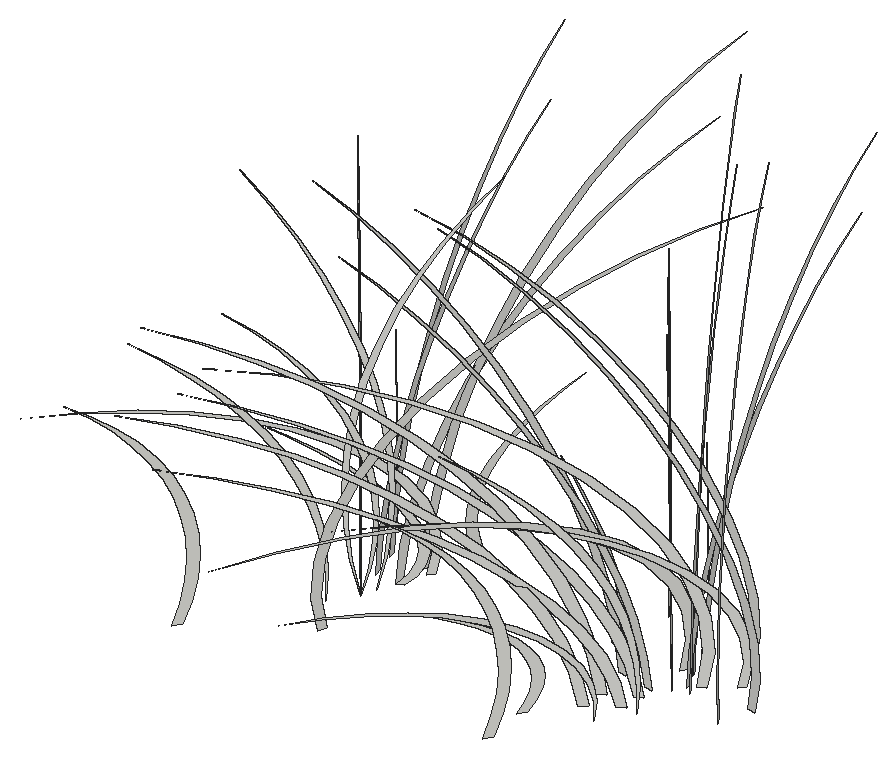
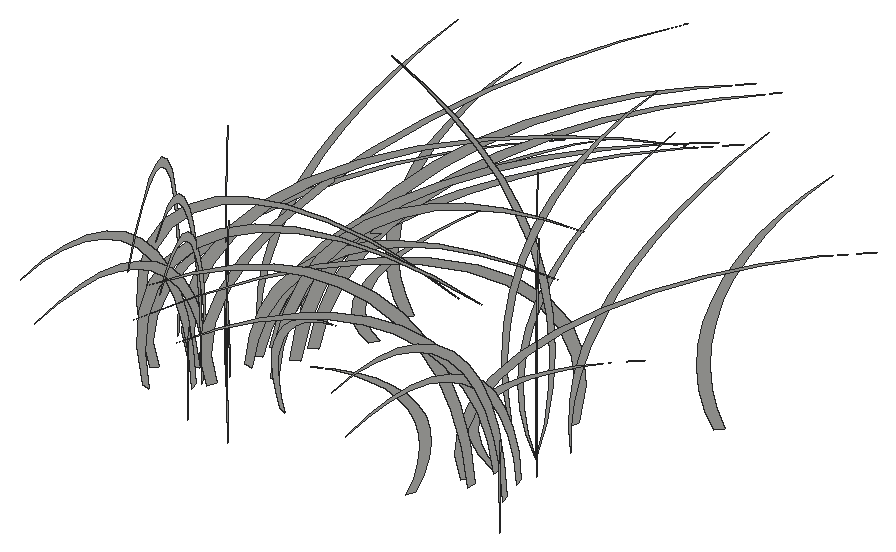
# SketchUp Ruby script. Lengths in inches.
U = 1.inch
M = Sketchup.active_model
def pt(a) = Geom::Point3d.new(a.map { |v| v * U })
def face(e, loops, mat)
  f = e.add_face(loops[0].map { |a| pt(a) })
  loops[1..].each { |l| e.add_face(l.map { |a| pt(a) }).erase! }
  f.material = f.back_material = mat if mat
  f
end
# faces: each face lists its corners as indices into pts; further lists are holes
def faces(e, pts, list, mat = nil) = list.each { |f| face(e, (f[0].is_a?(Array) ? f : [f]).map { |l| l.map { |i| pts[i] } }, mat) }
# xy, xz, yz: faces in a plane at the given z, y or x. An outline is a flat list of corners, or four numbers for a rectangle; further outlines are holes
def ring(l) = l.size == 4 ? [[l[0], l[1]], [l[2], l[1]], [l[2], l[3]], [l[0], l[3]]] : l.each_slice(2).to_a
def flat(e, list, mat, &to3) = list.each { |f| face(e, (f[0].is_a?(Array) ? f : [f]).map { |l| ring(l).map { |u, v| to3.(u, v) } }, mat) }
def xy(e, z, list, mat = nil) = flat(e, list, mat) { |x, y| [x, y, z] }
def xz(e, y, list, mat = nil) = flat(e, list, mat) { |x, z| [x, y, z] }
def yz(e, x, list, mat = nil) = flat(e, list, mat) { |y, z| [x, y, z] }
def lines(e, pts, list) = list.each { |a, b| e.add_line(pt(pts[a]), pt(pts[b])) }
# prism: a flat outline (further loops are holes) pulled along v
def prism(e, loops, v, mat = nil)
  f = face(e, loops, mat); d = Geom::Vector3d.new(v.map { |x| x * U })
  f.pushpull(f.normal.samedirection?(d) ? d.length : -d.length)
end
def box(e, o, s, mat = nil) = prism(e, [[o, [o[0] + s[0], o[1], o[2]], [o[0] + s[0], o[1] + s[1], o[2]], [o[0], o[1] + s[1], o[2]]]], [0, 0, s[2]], mat)
def at(x, y, z, deg = 0) = Geom::Transformation.translation(pt([x, y, z])) * Geom::Transformation.rotation(ORIGIN, Z_AXIS, deg.degrees)
def axes(o, x, y, z) = Geom::Transformation.new([*x, 0, *y, 0, *z, 0, *pt(o).to_a, 1])
def part(name) = M.definitions.add(name)
# library, detail: a bought-in or finely detailed component or shape, given as its bounding box
def library(name, o, s) = part(name).tap { |d| box(d.entities, o, s) }
def detail(e, o, s) = box(e.add_group.entities, o, s)
def put(e, d, t, mat = nil) = e.add_instance(d, t).tap { |i| i.material = mat if mat }
def group(e, t, mat = nil) = e.add_group.tap { |g| g.transformation = t; g.material = mat if mat }.entities
root = M.entities
g1 = group(root,at(473.71,252.72,0))
p = [[-3.94,-6,13.62],[-3.22,-4.9,12.76],[-2.57,-3.91,11.81],[-2,-3.04,10.79],[-1.5,-2.28,9.7],[-1.09,-1.66,8.57],
  [-0.77,-1.17,7.38],[-0.54,-0.83,6.17],[-0.41,-0.62,4.93],[-0.37,-0.5625,3.6875],[-0.43,-0.65,2.44],[-0.58,-0.88,1.21],
  [-0.83,-1.26,0],[-0.51,-0.77,0],[-0.23,-0.36,1.22],[-0.0625,-0.1,2.48],[0,0,3.75],[-0.04,-0.07,5.02],
  [-0.19,-0.29,6.28],[-0.45,-0.68,7.51],[-0.8,-1.22,8.7],[-1.26,-1.91,9.84],[-1.81,-2.75,10.91],[-2.44,-3.71,11.9],
  [-3.16,-4.8,12.8125]]
faces(g1,p,[[0,1,2,3,4,5,6,7,8,9,10,11,12,13,14,15,16,17,18,19,20,21,22,23,24]])
g2 = group(root,at(480.18,264.14,0))
p = [[-0.5,-0.57,0],[-0.22,-0.25,0],[0,0,1.46],[-0.09,-0.1,2.93],[-0.49,-0.56,4.375],[-1.19,-1.35,5.75],
  [-2.17,-2.47,7.03],[-3.41,-3.89,8.18],[-4.88,-5.56,9.17],[-6.54,-7.45,9.98],[-8.36,-9.51,10.58],[-10.27,-11.69,10.97],
  [-12.24,-13.9375,11.125],[-14.23,-16.19,11.05],[-12.28,-13.98,11.0625],[-10.36,-11.79,10.86],[-8.5,-9.67,10.44],[-6.74,-7.67,9.82],
  [-5.13,-5.84,9.01],[-3.71,-4.22,8.02],[-2.51,-2.85,6.89],[-1.54,-1.76,5.64],[-0.85,-0.97,4.29],[-0.44,-0.5,2.88],
  [-0.32,-0.37,1.4375]]
faces(g2,p,[[0,1,2,3,4,5,6,7,8,9,10,11,12,13,14,15,16,17,18,19,20,21,22,23,24]])
g3 = group(root,at(480.18,264.14,0))
p = [[-0.5,-0.57,0],[-0.22,-0.25,0],[0,0,1.46],[-0.09,-0.1,2.93],[-0.49,-0.56,4.375],[-1.19,-1.35,5.75],
  [-2.17,-2.47,7.03],[-3.41,-3.89,8.18],[-4.88,-5.56,9.17],[-6.54,-7.45,9.98],[-8.36,-9.51,10.58],[-10.27,-11.69,10.97],
  [-12.24,-13.9375,11.125],[-14.23,-16.19,11.05],[-12.28,-13.98,11.0625],[-10.36,-11.79,10.86],[-8.5,-9.67,10.44],[-6.74,-7.67,9.82],
  [-5.13,-5.84,9.01],[-3.71,-4.22,8.02],[-2.51,-2.85,6.89],[-1.54,-1.76,5.64],[-0.85,-0.97,4.29],[-0.44,-0.5,2.88],
  [-0.32,-0.37,1.4375]]
faces(g3,p,[[0,1,2,3,4,5,6,7,8,9,10,11,12,13,14,15,16,17,18,19,20,21,22,23,24]])
g4 = group(root,at(477.07,263.82,0))
p = [[-6.07,19.87,18.05],[-6.99,22.87,18.53],[-6.1,19.96,17.95],[-5.25,17.16,17.15],[-4.43,14.49,16.14],[-3.66,11.97,14.93],
  [-2.95,9.65,13.53],[-2.31,7.54,11.96],[-1.73,5.67,10.23],[-1.24,4.06,8.37],[-0.83,2.72,6.39],[-0.51,1.68,4.32],
  [-0.29,0.94,2.18],[-0.16,0.52,0],[0,0,0],[-0.11,0.35,2.23],[-0.32,1.04,4.43],[-0.63,2.07,6.55],
  [-1.04,3.41,8.57],[-1.55,5.05,10.47],[-2.13,6.98,12.22],[-2.8,9.16,13.8],[-3.54,11.58,15.1875],[-4.34,14.1875,16.37],
  [-5.1875,16.96,17.33]]
faces(g4,p,[[0,1,2,3,4,5,6,7,8,9,10,11,12,13,14,15,16,17,18,19,20,21,22,23,24]])
g5 = group(root,at(476.01,265.76,0))
p = [[-4.56,5.55,7.88],[-3.72,4.53,7.38],[-2.97,3.62,6.83],[-2.31,2.81,6.24],[-1.73,2.11,5.62],[-1.26,1.54,4.96],
  [-0.89,1.09,4.27],[-0.63,0.76,3.57],[-0.47,0.58,2.86],[-0.43,0.52,2.13],[-0.49,0.6,1.41],[-0.67,0.81,0.7],
  [-0.95,1.16,0],[-0.59,0.71,0],[-0.27,0.33,0.71],[-0.07,0.09,1.43],[0,0,2.17],[-0.05,0.0625,2.9],
  [-0.22,0.27,3.63],[-0.52,0.63,4.34],[-0.93,1.13,5.03],[-1.45,1.77,5.69],[-2.09,2.54,6.3125],[-2.82,3.43,6.89],
  [-3.65,4.44,7.41]]
faces(g5,p,[[0,1,2,3,4,5,6,7,8,9,10,11,12,13,14,15,16,17,18,19,20,21,22,23,24]])
g6 = group(root,at(477.3,261.15,0))
p = [[-6.74,8.21,19.61],[-5.67,6.9,18.16],[-4.68,5.7,16.67],[-3.78,4.6,15.125],[-2.98,3.62,13.55],[-2.27,2.76,11.93],
  [-1.65,2.01,10.28],[-1.14,1.39,8.61],[-0.72,0.88,6.91],[-0.41,0.5,5.2],[-0.2,0.24,3.47],[-0.09,0.11,1.74],
  [-0.09,0.11,0],[0,0,1.74],[-0.03,0.04,3.49],[-0.1875,0.23,5.23],[-0.46,0.56,6.96],[-0.85,1.04,8.67],
  [-1.36,1.66,10.36],[-1.98,2.42,12.01],[-2.72,3.3125,13.63],[-3.57,4.35,15.21],[-4.52,5.51,16.73],[-5.58,6.8,18.2]]
faces(g6,p,[[0,1,2,3,4,5,6,7,8,9,10,11,12,13,14,15,16,17,18,19,20,21,22,23]])
g7 = group(root,at(477.3,261.15,0))
p = [[-6.74,8.21,19.61],[-5.67,6.9,18.16],[-4.68,5.7,16.67],[-3.78,4.6,15.125],[-2.98,3.62,13.55],[-2.27,2.76,11.93],
  [-1.65,2.01,10.28],[-1.14,1.39,8.61],[-0.72,0.88,6.91],[-0.41,0.5,5.2],[-0.2,0.24,3.47],[-0.09,0.11,1.74],
  [-0.09,0.11,0],[0,0,1.74],[-0.03,0.04,3.49],[-0.1875,0.23,5.23],[-0.46,0.56,6.96],[-0.85,1.04,8.67],
  [-1.36,1.66,10.36],[-1.98,2.42,12.01],[-2.72,3.3125,13.63],[-3.57,4.35,15.21],[-4.52,5.51,16.73],[-5.58,6.8,18.2]]
faces(g7,p,[[0,1,2,3,4,5,6,7,8,9,10,11,12,13,14,15,16,17,18,19,20,21,22,23]])
g8 = group(root,at(477.64,261.97,0))
p = [[-6.07,19.87,14.56],[-6.99,22.87,14.94],[-6.1,19.96,14.48],[-5.25,17.16,13.83],[-4.43,14.49,13.02],[-3.66,11.97,12.04],
  [-2.95,9.65,10.91],[-2.31,7.54,9.64],[-1.73,5.67,8.25],[-1.24,4.06,6.75],[-0.83,2.72,5.15],[-0.51,1.68,3.49],
  [-0.29,0.94,1.76],[-0.16,0.52,0],[0,0,0],[-0.11,0.35,1.8],[-0.32,1.04,3.57],[-0.63,2.07,5.28],
  [-1.04,3.41,6.91],[-1.55,5.05,8.44],[-2.13,6.98,9.85],[-2.8,9.16,11.13],[-3.54,11.58,12.25],[-4.34,14.1875,13.2],
  [-5.1875,16.96,13.97]]
faces(g8,p,[[0,1,2,3,4,5,6,7,8,9,10,11,12,13,14,15,16,17,18,19,20,21,22,23,24]])
g9 = group(root,at(477.44,258.4,0))
p = [[-5.83,-8.875,16.67],[-4.9,-7.46,15.44],[-4.05,-6.16,14.17],[-3.27,-4.98,12.86],[-2.58,-3.92,11.51],[-1.96,-2.98,10.14],
  [-1.43,-2.18,8.74],[-0.99,-1.5,7.31],[-0.63,-0.95,5.87],[-0.36,-0.54,4.42],[-0.17,-0.26,2.95],[-0.08,-0.12,1.48],
  [-0.08,-0.12,0],[0,0,1.48],[-0.03,-0.04,2.97],[-0.16,-0.24,4.45],[-0.4,-0.6,5.92],[-0.74,-1.12,7.37],
  [-1.18,-1.79,8.81],[-1.72,-2.61,10.21],[-2.36,-3.58,11.59],[-3.09,-4.7,12.93],[-3.92,-5.96,14.22],[-4.83,-7.35,15.47]]
faces(g9,p,[[0,1,2,3,4,5,6,7,8,9,10,11,12,13,14,15,16,17,18,19,20,21,22,23]])
g10 = group(root,at(479.55,261.125,0))
p = [[-0.89,-0.32,0],[-0.4,-0.14,1.97],[-0.1,-0.04,3.96],[0,0,5.95],[-0.1,-0.03,7.95],[-0.39,-0.14,9.9375],
  [-0.89,-0.3125,11.91],[-1.57,-0.56,13.85],[-2.45,-0.87,15.76],[-3.52,-1.25,17.63],[-4.77,-1.6875,19.44],[-6.19,-2.19,21.2],
  [-7.79,-2.76,22.89],[-6.29,-2.23,21.17],[-4.94,-1.75,19.4],[-3.76,-1.33,17.58],[-2.74,-0.97,15.71],[-1.89,-0.67,13.8],
  [-1.22,-0.43,11.86],[-0.72,-0.25,9.9],[-0.4,-0.14,7.93],[-0.25,-0.09,5.94],[-0.29,-0.1,3.95],[-0.5,-0.18,1.97]]
faces(g10,p,[[0,1,2,3,4,5,6,7,8,9,10,11,12,13,14,15,16,17,18,19,20,21,22,23]])
g11 = group(root,at(480.65,262.48,0))
p = [[-9.01,-2.98,7.88],[-7.3,-2.41,7.38],[-5.75,-1.9,6.83],[-4.38,-1.45,6.24],[-3.2,-1.06,5.62],[-2.23,-0.74,4.96],
  [-1.47,-0.49,4.27],[-0.92,-0.31,3.57],[-0.61,-0.2,2.86],[-0.51,-0.17,2.13],[-0.65,-0.21,1.41],[-1.01,-0.33,0.7],
  [-1.6,-0.53,0],[-1.21,-0.4,0],[-0.54,-0.18,0.69],[-0.12,-0.04,1.4],[0.06,0.02,2.13],[-0.02,-0.01,2.85],
  [-0.35,-0.11,3.58],[-0.92,-0.3,4.29],[-1.73,-0.57,4.98],[-2.78,-0.92,5.64],[-4.05,-1.34,6.27],[-5.52,-1.82,6.86],
  [-7.18,-2.375,7.4]]
faces(g11,p,[[0,1,2,3,4,5,6,7,8,9,10,11,12,13,14,15,16,17,18,19,20,21,22,23,24]])
g12 = group(root,at(478.99,259.1,0))
p = [[-0.6,0.73,0],[-0.27,0.33,1.77],[-0.07,0.08,3.57],[0,0,5.36],[-0.07,0.08,7.16],[-0.27,0.32,8.95],
  [-0.6,0.73,10.73],[-1.06,1.29,12.48],[-1.65,2.01,14.2],[-2.37,2.88,15.88],[-3.21,3.91,17.52],[-4.17,5.08,19.1],
  [-5.25,6.39,20.625],[-4.23,5.15,19.08],[-3.33,4.05,17.48],[-2.53,3.08,15.83],[-1.84,2.25,14.15],[-1.27,1.55,12.43],
  [-0.82,1,10.6875],[-0.48,0.59,8.92],[-0.27,0.32,7.14],[-0.17,0.21,5.35],[-0.19,0.24,3.5625],[-0.34,0.41,1.78]]
faces(g12,p,[[0,1,2,3,4,5,6,7,8,9,10,11,12,13,14,15,16,17,18,19,20,21,22,23]])
g13 = group(root,at(478.9,260.62,0))
p = [[-0.52,-0.79,0],[-0.23,-0.35,1.51],[-0.06,-0.09,3.03],[0,0,4.56],[-0.06,-0.09,6.09],[-0.23,-0.35,7.61],
  [-0.52,-0.79,9.12],[-0.92,-1.39,10.61],[-1.43,-2.17,12.07],[-2.05,-3.12,13.5],[-2.78,-4.23,14.89],[-3.61,-5.49,16.24],
  [-4.54,-6.91,17.53],[-3.66,-5.57,16.21],[-2.88,-4.38,14.86],[-2.1875,-3.33,13.46],[-1.6,-2.43,12.03],[-1.1,-1.68,10.57],
  [-0.71,-1.08,9.08],[-0.42,-0.64,7.58],[-0.23,-0.35,6.07],[-0.15,-0.22,4.55],[-0.17,-0.25,3.03],[-0.29,-0.44,1.51]]
faces(g13,p,[[0,1,2,3,4,5,6,7,8,9,10,11,12,13,14,15,16,17,18,19,20,21,22,23]])
g14 = group(root,at(479.01,261.85,0))
p = [[1.63,20.71,16.73],[1.875,23.84,17.17],[1.64,20.8125,16.64],[1.41,17.89,15.9],[1.1875,15.1,14.96],[0.98,12.48,13.84],
  [0.79,10.06,12.54],[0.62,7.86,11.08],[0.47,5.91,9.48],[0.33,4.23,7.76],[0.22,2.84,5.92],[0.14,1.75,4.01],
  [0.08,0.98,2.02],[0.04,0.54,0],[0,0,0],[0.03,0.36,2.07],[0.09,1.09,4.1],[0.17,2.15,6.07],
  [0.28,3.55,7.94],[0.41,5.27,9.7],[0.57,7.28,11.33],[0.75,9.55,12.79],[0.95,12.07,14.08],[1.16,14.79,15.17],
  [1.39,17.68,16.0625]]
faces(g14,p,[[0,1,2,3,4,5,6,7,8,9,10,11,12,13,14,15,16,17,18,19,20,21,22,23,24]])
g15 = group(root,at(479.16,263.78,0))
p = [[1.63,20.71,20.75],[1.875,23.84,21.3],[1.64,20.8125,20.63],[1.41,17.89,19.72],[1.1875,15.1,18.55],[0.98,12.48,17.16],
  [0.79,10.06,15.55],[0.62,7.86,13.74],[0.47,5.91,11.76],[0.33,4.23,9.62],[0.22,2.84,7.35],[0.14,1.75,4.97],
  [0.08,0.98,2.51],[0.04,0.54,0],[0,0,0],[0.03,0.36,2.57],[0.09,1.09,5.09],[0.17,2.15,7.53],
  [0.28,3.55,9.85],[0.41,5.27,12.03],[0.57,7.28,14.04],[0.75,9.55,15.86],[0.95,12.07,17.46],[1.16,14.79,18.82],
  [1.39,17.68,19.92]]
faces(g15,p,[[0,1,2,3,4,5,6,7,8,9,10,11,12,13,14,15,16,17,18,19,20,21,22,23,24]])
g16 = group(root,at(477.71,259.16,0))
p = [[0.67,0.67,0],[0.3,0.3,2.04],[0.08,0.08,4.1],[0,0,6.17],[0.07,0.07,8.23],[0.3,0.3,10.29],
  [0.66,0.66,12.33],[1.18,1.18,14.34],[1.84,1.84,16.32],[2.64,2.64,18.26],[3.58,3.58,20.14],[4.65,4.65,21.96],
  [5.84,5.84,23.71],[4.72,4.72,21.93],[3.71,3.71,20.09],[2.82,2.82,18.2],[2.05,2.05,16.26],[1.42,1.42,14.29],
  [0.91,0.91,12.29],[0.54,0.54,10.26],[0.3,0.3,8.21],[0.1875,0.1875,6.15],[0.22,0.22,4.09],[0.375,0.375,2.04]]
faces(g16,p,[[0,1,2,3,4,5,6,7,8,9,10,11,12,13,14,15,16,17,18,19,20,21,22,23]])
g17 = group(root,at(480.7,265.375,0))
p = [[2.34,6.79,9.0625],[1.91,5.55,8.49],[1.52,4.43,7.85],[1.18,3.44,7.18],[0.89,2.58,6.45],[0.65,1.88,5.7],
  [0.46,1.33,4.91],[0.32,0.93,4.1],[0.24,0.7,3.28],[0.22,0.64,2.45],[0.25,0.74,1.625],[0.34,1,0.8],
  [0.49,1.42,0],[0.3,0.875,0],[0.14,0.4,0.81],[0.04,0.11,1.65],[0,0,2.49],[0.03,0.07,3.34],
  [0.11,0.33,4.17],[0.27,0.77,4.99],[0.48,1.38,5.79],[0.75,2.17,6.54],[1.07,3.11,7.26],[1.45,4.2,7.92],
  [1.87,5.43,8.52]]
faces(g17,p,[[0,1,2,3,4,5,6,7,8,9,10,11,12,13,14,15,16,17,18,19,20,21,22,23,24]])
g18 = group(root,at(494,261.72,0))
p = [[-20.46,3.64,18.05],[-23.54,4.19,18.53],[-20.55,3.66,17.95],[-17.67,3.15,17.15],[-14.91,2.66,16.14],[-12.33,2.2,14.93],
  [-9.93,1.77,13.53],[-7.76,1.38,11.96],[-5.84,1.04,10.23],[-4.18,0.74,8.37],[-2.8,0.5,6.39],[-1.73,0.31,4.32],
  [-0.97,0.17,2.18],[-0.53,0.09,0],[0,0,0],[-0.36,0.0625,2.23],[-1.07,0.19,4.43],[-2.125,0.38,6.55],
  [-3.51,0.625,8.57],[-5.2,0.93,10.47],[-7.1875,1.28,12.22],[-9.43,1.68,13.8],[-11.92,2.125,15.1875],[-14.61,2.6,16.37],
  [-17.46,3.11,17.33]]
faces(g18,p,[[0,1,2,3,4,5,6,7,8,9,10,11,12,13,14,15,16,17,18,19,20,21,22,23,24]])
g19 = group(root,at(478.86,255.22,0))
p = [[0.26,0.96,0],[0.11,0.43,0],[0,0,2.01],[0.05,0.17,4.04],[0.25,0.9375,6.02],[0.62,2.28,7.92],
  [1.125,4.16,9.68],[1.76,6.54,11.26],[2.52,9.35,12.62],[3.38,12.53,13.73],[4.32,16,14.5625],[5.31,19.67,15.09],
  [6.33,23.45,15.31],[7.35,27.24,15.2],[6.35,23.52,15.22],[5.35,19.83,14.94],[4.39,16.27,14.37],[3.48,12.91,13.51],
  [2.65,9.83,12.39],[1.92,7.11,11.04],[1.29,4.8,9.48],[0.8,2.96,7.75],[0.44,1.63,5.9],[0.23,0.84,3.96],
  [0.17,0.62,1.98]]
faces(g19,p,[[0,1,2,3,4,5,6,7,8,9,10,11,12,13,14,15,16,17,18,19,20,21,22,23,24]])
g20 = group(root,at(494.4,259.62,0))
p = [[-18.45,-9.5625,18.05],[-21.23,-11,18.53],[-18.53,-9.61,17.95],[-15.93,-8.26,17.15],[-13.45,-6.97,16.14],[-11.12,-5.76,14.93],
  [-8.96,-4.64,13.53],[-7,-3.63,11.96],[-5.26,-2.73,10.23],[-3.77,-1.95,8.37],[-2.53,-1.3125,6.39],[-1.5625,-0.81,4.32],
  [-0.875,-0.45,2.18],[-0.48,-0.25,0],[0,0,0],[-0.32,-0.17,2.23],[-0.97,-0.5,4.43],[-1.92,-0.99,6.55],
  [-3.16,-1.64,8.57],[-4.69,-2.43,10.47],[-6.48,-3.36,12.22],[-8.51,-4.41,13.8],[-10.75,-5.57,15.1875],[-13.17,-6.83,16.37],
  [-15.75,-8.16,17.33]]
faces(g20,p,[[0,1,2,3,4,5,6,7,8,9,10,11,12,13,14,15,16,17,18,19,20,21,22,23,24]])
g21 = group(root,at(494.4,259.62,0))
p = [[-18.45,-9.5625,18.05],[-21.23,-11,18.53],[-18.53,-9.61,17.95],[-15.93,-8.26,17.15],[-13.45,-6.97,16.14],[-11.12,-5.76,14.93],
  [-8.96,-4.64,13.53],[-7,-3.63,11.96],[-5.26,-2.73,10.23],[-3.77,-1.95,8.37],[-2.53,-1.3125,6.39],[-1.5625,-0.81,4.32],
  [-0.875,-0.45,2.18],[-0.48,-0.25,0],[0,0,0],[-0.32,-0.17,2.23],[-0.97,-0.5,4.43],[-1.92,-0.99,6.55],
  [-3.16,-1.64,8.57],[-4.69,-2.43,10.47],[-6.48,-3.36,12.22],[-8.51,-4.41,13.8],[-10.75,-5.57,15.1875],[-13.17,-6.83,16.37],
  [-15.75,-8.16,17.33]]
faces(g21,p,[[0,1,2,3,4,5,6,7,8,9,10,11,12,13,14,15,16,17,18,19,20,21,22,23,24]])
g22 = group(root,at(495.91,261.38,0))
p = [[-20.46,3.64,14.56],[-23.54,4.19,14.94],[-20.55,3.66,14.48],[-17.67,3.15,13.83],[-14.91,2.66,13.02],[-12.33,2.2,12.04],
  [-9.93,1.77,10.91],[-7.76,1.38,9.64],[-5.84,1.04,8.25],[-4.18,0.74,6.75],[-2.8,0.5,5.15],[-1.73,0.31,3.49],
  [-0.97,0.17,1.76],[-0.53,0.09,0],[0,0,0],[-0.36,0.0625,1.8],[-1.07,0.19,3.57],[-2.125,0.38,5.28],
  [-3.51,0.625,6.91],[-5.2,0.93,8.44],[-7.1875,1.28,9.85],[-9.43,1.68,11.13],[-11.92,2.125,12.25],[-14.61,2.6,13.2],
  [-17.46,3.11,13.97]]
faces(g22,p,[[0,1,2,3,4,5,6,7,8,9,10,11,12,13,14,15,16,17,18,19,20,21,22,23,24]])
g23 = group(root,at(494.44,258.13,0))
p = [[-17.17,-11.7,15.34],[-19.76,-13.47,15.75],[-17.25,-11.76,15.26],[-14.83,-10.11,14.58],[-12.52,-8.53,13.72],[-10.35,-7.05,12.69],
  [-8.34,-5.68,11.5],[-6.52,-4.44,10.16],[-4.9,-3.34,8.7],[-3.51,-2.39,7.11],[-2.35,-1.6,5.43],[-1.45,-0.99,3.67],
  [-0.82,-0.56,1.86],[-0.45,-0.3,0],[0,0,0],[-0.3,-0.21,1.9],[-0.9,-0.61,3.76],[-1.78,-1.22,5.57],
  [-2.95,-2.01,7.28],[-4.37,-2.98,8.9],[-6.03,-4.11,10.39],[-7.92,-5.4,11.73],[-10,-6.82,12.91],[-12.26,-8.36,13.91],
  [-14.66,-9.99,14.73]]
faces(g23,p,[[0,1,2,3,4,5,6,7,8,9,10,11,12,13,14,15,16,17,18,19,20,21,22,23,24]])
g24 = group(root,at(496.11,260.51,0))
p = [[-18.45,-9.5625,14.56],[-21.23,-11,14.94],[-18.53,-9.61,14.48],[-15.93,-8.26,13.83],[-13.45,-6.97,13.02],[-11.12,-5.76,12.04],
  [-8.96,-4.64,10.91],[-7,-3.63,9.64],[-5.26,-2.73,8.25],[-3.77,-1.95,6.75],[-2.53,-1.3125,5.15],[-1.5625,-0.81,3.49],
  [-0.875,-0.45,1.76],[-0.48,-0.25,0],[0,0,0],[-0.32,-0.17,1.8],[-0.97,-0.5,3.57],[-1.92,-0.99,5.28],
  [-3.16,-1.64,6.91],[-4.69,-2.43,8.44],[-6.48,-3.36,9.85],[-8.51,-4.41,11.13],[-10.75,-5.57,12.25],[-13.17,-6.83,13.2],
  [-15.75,-8.16,13.97]]
faces(g24,p,[[0,1,2,3,4,5,6,7,8,9,10,11,12,13,14,15,16,17,18,19,20,21,22,23,24]])
g25 = group(root,at(496.11,260.51,0))
p = [[-18.45,-9.5625,14.56],[-21.23,-11,14.94],[-18.53,-9.61,14.48],[-15.93,-8.26,13.83],[-13.45,-6.97,13.02],[-11.12,-5.76,12.04],
  [-8.96,-4.64,10.91],[-7,-3.63,9.64],[-5.26,-2.73,8.25],[-3.77,-1.95,6.75],[-2.53,-1.3125,5.15],[-1.5625,-0.81,3.49],
  [-0.875,-0.45,1.76],[-0.48,-0.25,0],[0,0,0],[-0.32,-0.17,1.8],[-0.97,-0.5,3.57],[-1.92,-0.99,5.28],
  [-3.16,-1.64,6.91],[-4.69,-2.43,8.44],[-6.48,-3.36,9.85],[-8.51,-4.41,11.13],[-10.75,-5.57,12.25],[-13.17,-6.83,13.2],
  [-15.75,-8.16,13.97]]
faces(g25,p,[[0,1,2,3,4,5,6,7,8,9,10,11,12,13,14,15,16,17,18,19,20,21,22,23,24]])
g26 = group(root,at(498.98,266.23,0))
p = [[-0.91,0.16,0],[-0.4,0.07,0],[0,0,2.0625],[-0.16,0.03,4.13],[-0.89,0.16,6.16],[-2.17,0.39,8.1],
  [-3.95,0.7,9.91],[-6.21,1.11,11.52],[-8.88,1.58,12.92],[-11.91,2.12,14.05],[-15.2,2.71,14.9],[-18.68,3.33,15.45],
  [-22.27,3.97,15.67],[-25.88,4.61,15.5625],[-22.34,3.98,15.58],[-18.84,3.36,15.29],[-15.45,2.75,14.71],[-12.26,2.18,13.83],
  [-9.34,1.66,12.68],[-6.75,1.2,11.3],[-4.56,0.8125,9.7],[-2.81,0.5,7.9375],[-1.55,0.28,6.04],[-0.8,0.14,4.05],
  [-0.59,0.1,2.02]]
faces(g26,p,[[0,1,2,3,4,5,6,7,8,9,10,11,12,13,14,15,16,17,18,19,20,21,22,23,24]])
g27 = group(root,at(498.98,266.23,0))
p = [[-0.91,0.16,0],[-0.4,0.07,0],[0,0,2.0625],[-0.16,0.03,4.13],[-0.89,0.16,6.16],[-2.17,0.39,8.1],
  [-3.95,0.7,9.91],[-6.21,1.11,11.52],[-8.88,1.58,12.92],[-11.91,2.12,14.05],[-15.2,2.71,14.9],[-18.68,3.33,15.45],
  [-22.27,3.97,15.67],[-25.88,4.61,15.5625],[-22.34,3.98,15.58],[-18.84,3.36,15.29],[-15.45,2.75,14.71],[-12.26,2.18,13.83],
  [-9.34,1.66,12.68],[-6.75,1.2,11.3],[-4.56,0.8125,9.7],[-2.81,0.5,7.9375],[-1.55,0.28,6.04],[-0.8,0.14,4.05],
  [-0.59,0.1,2.02]]
faces(g27,p,[[0,1,2,3,4,5,6,7,8,9,10,11,12,13,14,15,16,17,18,19,20,21,22,23,24]])
g28 = group(root,at(496.04,259.22,0))
p = [[-17.17,-11.7,12.375],[-19.76,-13.47,12.7],[-17.25,-11.76,12.31],[-14.83,-10.11,11.76],[-12.52,-8.53,11.07],[-10.35,-7.05,10.23],
  [-8.34,-5.68,9.27],[-6.52,-4.44,8.2],[-4.9,-3.34,7.01],[-3.51,-2.39,5.74],[-2.35,-1.6,4.38],[-1.45,-0.99,2.96],
  [-0.82,-0.56,1.5],[-0.45,-0.3,0],[0,0,0],[-0.3,-0.21,1.53],[-0.9,-0.61,3.03],[-1.78,-1.22,4.49],
  [-2.95,-2.01,5.875],[-4.37,-2.98,7.18],[-6.03,-4.11,8.375],[-7.92,-5.4,9.46],[-10,-6.82,10.41],[-12.26,-8.36,11.22],
  [-14.66,-9.99,11.88]]
faces(g28,p,[[0,1,2,3,4,5,6,7,8,9,10,11,12,13,14,15,16,17,18,19,20,21,22,23,24]])
g29 = group(root,at(498.24,263.54,0))
p = [[-0.82,-0.43,0],[-0.36,-0.1875,0],[0,0,2.0625],[-0.15,-0.08,4.13],[-0.8,-0.42,6.16],[-1.95,-1.01,8.1],
  [-3.57,-1.85,9.91],[-5.6,-2.9,11.52],[-8.01,-4.15,12.92],[-10.74,-5.57,14.05],[-13.71,-7.1,14.9],[-16.85,-8.73,15.45],
  [-20.09,-10.41,15.67],[-23.34,-12.1,15.5625],[-20.15,-10.44,15.58],[-16.99,-8.81,15.29],[-13.9375,-7.22,14.71],[-11.06,-5.73,13.83],
  [-8.42,-4.37,12.68],[-6.09,-3.16,11.3],[-4.11,-2.13,9.7],[-2.53,-1.3125,7.9375],[-1.4,-0.72,6.04],[-0.72,-0.375,4.05],
  [-0.53,-0.27,2.02]]
faces(g29,p,[[0,1,2,3,4,5,6,7,8,9,10,11,12,13,14,15,16,17,18,19,20,21,22,23,24]])
g30 = group(root,at(501.83,262.67,0))
p = [[-0.95,0.28,0],[-0.42,0.125,0],[0,0,2.01],[-0.17,0.05,4.04],[-0.93,0.27,6.02],[-2.27,0.66,7.92],
  [-4.14,1.21,9.68],[-6.5,1.9,11.26],[-9.3,2.72,12.62],[-12.46,3.64,13.73],[-15.91,4.65,14.5625],[-19.55,5.72,15.09],
  [-23.3125,6.82,15.31],[-27.08,7.92,15.2],[-23.38,6.84,15.22],[-19.72,5.77,14.94],[-16.17,4.73,14.37],[-12.83,3.75,13.51],
  [-9.77,2.86,12.39],[-7.0625,2.07,11.04],[-4.77,1.39,9.48],[-2.94,0.86,7.75],[-1.62,0.47,5.9],[-0.84,0.25,3.96],
  [-0.61,0.18,1.98]]
faces(g30,p,[[0,1,2,3,4,5,6,7,8,9,10,11,12,13,14,15,16,17,18,19,20,21,22,23,24]])
g31 = group(root,at(492.5625,263.42,0))
p = [[-6.53,2.99,7.88],[-5.33,2.44,7.38],[-4.26,1.95,6.83],[-3.3,1.51,6.24],[-2.48,1.14,5.62],[-1.81,0.83,4.96],
  [-1.28,0.58,4.27],[-0.9,0.41,3.57],[-0.68,0.31,2.86],[-0.61,0.28,2.13],[-0.71,0.32,1.41],[-0.96,0.4375,0.7],
  [-1.37,0.625,0],[-0.84,0.38,0],[-0.39,0.18,0.71],[-0.11,0.05,1.43],[0,0,2.17],[-0.07,0.03,2.9],
  [-0.32,0.15,3.63],[-0.74,0.34,4.34],[-1.33,0.61,5.03],[-2.08,0.95,5.69],[-2.99,1.37,6.3125],[-4.04,1.85,6.89],
  [-5.22,2.39,7.41]]
faces(g31,p,[[0,1,2,3,4,5,6,7,8,9,10,11,12,13,14,15,16,17,18,19,20,21,22,23,24]])
g32 = group(root,at(495.33,263.65,0))
p = [[-10.66,12.98,9.9],[-9.23,11.23,9.83],[-7.82,9.52,9.59],[-6.46,7.86,9.18],[-5.18,6.3,8.61],[-3.99,4.86,7.88],
  [-2.93,3.57,7.02],[-2.02,2.46,6.03],[-1.27,1.54,4.95],[-0.6875,0.84,3.78],[-0.29,0.36,2.55],[-0.1,0.12,1.28],
  [-0.09,0.12,0],[0,0,1.3],[-0.125,0.15,2.61],[-0.47,0.57,3.875],[-1.02,1.24,5.09],[-1.77,2.15,6.21],
  [-2.69,3.28,7.22],[-3.78,4.6,8.1],[-5,6.09,8.82],[-6.33,7.71,9.37],[-7.74,9.43,9.74],[-9.2,11.19,9.92]]
faces(g32,p,[[0,1,2,3,4,5,6,7,8,9,10,11,12,13,14,15,16,17,18,19,20,21,22,23]])
g33 = group(root,at(496.58,263.92,0))
p = [[-11.32,17.43,20.75],[-13.02,20.05,21.3],[-11.37,17.51,20.63],[-9.77,15.05,19.72],[-8.25,12.7,18.55],[-6.82,10.5,17.16],
  [-5.5,8.46,15.55],[-4.29,6.61,13.74],[-3.23,4.97,11.76],[-2.3125,3.56,9.62],[-1.55,2.39,7.35],[-0.96,1.47,4.97],
  [-0.54,0.83,2.51],[-0.29,0.45,0],[0,0,0],[-0.2,0.31,2.57],[-0.59,0.91,5.09],[-1.18,1.8125,7.53],
  [-1.94,2.99,9.85],[-2.88,4.43,12.03],[-3.98,6.12,14.04],[-5.22,8.04,15.86],[-6.59,10.15,17.46],[-8.08,12.44,18.82],
  [-9.66,14.88,19.92]]
faces(g33,p,[[0,1,2,3,4,5,6,7,8,9,10,11,12,13,14,15,16,17,18,19,20,21,22,23,24]])
g34 = group(root,at(492.46,267.14,0))
p = [[-4.56,5.55,16.02],[-3.72,4.53,15.01],[-2.97,3.62,13.89],[-2.31,2.81,12.69],[-1.73,2.11,11.42],[-1.26,1.54,10.08],
  [-0.89,1.09,8.6875],[-0.63,0.76,7.26],[-0.47,0.58,5.8],[-0.43,0.52,4.34],[-0.49,0.6,2.87],[-0.67,0.81,1.42],
  [-0.95,1.16,0],[-0.59,0.71,0],[-0.27,0.33,1.44],[-0.07,0.09,2.92],[0,0,4.41],[-0.05,0.0625,5.9],
  [-0.22,0.27,7.38],[-0.52,0.63,8.83],[-0.93,1.13,10.23],[-1.45,1.77,11.57],[-2.09,2.54,12.83],[-2.82,3.43,14.01],
  [-3.65,4.44,15.07]]
faces(g34,p,[[0,1,2,3,4,5,6,7,8,9,10,11,12,13,14,15,16,17,18,19,20,21,22,23,24]])
g35 = group(root,at(492.46,267.14,0))
p = [[-4.56,5.55,16.02],[-3.72,4.53,15.01],[-2.97,3.62,13.89],[-2.31,2.81,12.69],[-1.73,2.11,11.42],[-1.26,1.54,10.08],
  [-0.89,1.09,8.6875],[-0.63,0.76,7.26],[-0.47,0.58,5.8],[-0.43,0.52,4.34],[-0.49,0.6,2.87],[-0.67,0.81,1.42],
  [-0.95,1.16,0],[-0.59,0.71,0],[-0.27,0.33,1.44],[-0.07,0.09,2.92],[0,0,4.41],[-0.05,0.0625,5.9],
  [-0.22,0.27,7.38],[-0.52,0.63,8.83],[-0.93,1.13,10.23],[-1.45,1.77,11.57],[-2.09,2.54,12.83],[-2.82,3.43,14.01],
  [-3.65,4.44,15.07]]
faces(g35,p,[[0,1,2,3,4,5,6,7,8,9,10,11,12,13,14,15,16,17,18,19,20,21,22,23,24]])
g36 = group(root,at(496.15,264.73,0))
p = [[-0.37,-0.92,0],[-0.16,-0.41,0],[0,0,1.75],[-0.07,-0.17,3.51],[-0.36,-0.9,5.24],[-0.88,-2.19,6.89],
  [-1.61,-4,8.42],[-2.53,-6.28,9.8],[-3.61,-8.99,10.98],[-4.84,-12.04,11.95],[-6.18,-15.375,12.67],[-7.6,-18.9,13.13],
  [-9.06,-22.53,13.32],[-10.53,-26.18,13.23],[-9.09,-22.6,13.25],[-7.66,-19.06,13],[-6.29,-15.63,12.5],[-4.99,-12.41,11.75],
  [-3.8,-9.45,10.78],[-2.75,-6.83,9.6],[-1.85,-4.61,8.25],[-1.14,-2.84,6.75],[-0.63,-1.57,5.13],[-0.33,-0.8125,3.44],
  [-0.24,-0.59,1.72]]
faces(g36,p,[[0,1,2,3,4,5,6,7,8,9,10,11,12,13,14,15,16,17,18,19,20,21,22,23,24]])
g37 = group(root,at(492.9,256.54,0))
p = [[-3.94,-6,6.7],[-3.22,-4.9,6.27],[-2.57,-3.91,5.81],[-2,-3.04,5.31],[-1.5,-2.28,4.77],[-1.09,-1.66,4.21],
  [-0.77,-1.17,3.63],[-0.54,-0.83,3.03],[-0.41,-0.62,2.43],[-0.37,-0.5625,1.8125],[-0.43,-0.65,1.2],[-0.58,-0.88,0.59],
  [-0.83,-1.26,0],[-0.51,-0.77,0],[-0.23,-0.36,0.6],[-0.0625,-0.1,1.22],[0,0,1.84],[-0.04,-0.07,2.47],
  [-0.19,-0.29,3.09],[-0.45,-0.68,3.69],[-0.8,-1.22,4.28],[-1.26,-1.91,4.84],[-1.81,-2.75,5.37],[-2.44,-3.71,5.86],
  [-3.16,-4.8,6.3]]
faces(g37,p,[[0,1,2,3,4,5,6,7,8,9,10,11,12,13,14,15,16,17,18,19,20,21,22,23,24]])
g38 = group(root,at(495.67,257.24,0))
p = [[-9.23,-14.04,8.41],[-7.99,-12.15,8.36],[-6.77,-10.29,8.15],[-5.59,-8.5,7.8],[-4.48,-6.8125,7.32],[-3.46,-5.26,6.7],
  [-2.54,-3.86,5.97],[-1.75,-2.66,5.13],[-1.09,-1.67,4.2],[-0.59,-0.9,3.21],[-0.25,-0.39,2.16],[-0.08,-0.125,1.09],
  [-0.08,-0.125,0],[0,0,1.11],[-0.11,-0.16,2.21],[-0.4,-0.61,3.29],[-0.88,-1.34,4.32],[-1.53,-2.33,5.28],
  [-2.33,-3.55,6.14],[-3.27,-4.98,6.88],[-4.33,-6.59,7.5],[-5.48,-8.34,7.97],[-6.7,-10.19,8.28],[-7.96,-12.11,8.43]]
faces(g38,p,[[0,1,2,3,4,5,6,7,8,9,10,11,12,13,14,15,16,17,18,19,20,21,22,23]])
g39 = group(root,at(497.63,262.3,0))
p = [[-11.32,17.43,16.73],[-13.02,20.05,17.17],[-11.37,17.51,16.64],[-9.77,15.05,15.9],[-8.25,12.7,14.96],[-6.82,10.5,13.84],
  [-5.5,8.46,12.54],[-4.29,6.61,11.08],[-3.23,4.97,9.48],[-2.3125,3.56,7.76],[-1.55,2.39,5.92],[-0.96,1.47,4.01],
  [-0.54,0.83,2.02],[-0.29,0.45,0],[0,0,0],[-0.2,0.31,2.07],[-0.59,0.91,4.1],[-1.18,1.8125,6.07],
  [-1.94,2.99,7.94],[-2.88,4.43,9.7],[-3.98,6.12,11.33],[-5.22,8.04,12.79],[-6.59,10.15,14.08],[-8.08,12.44,15.17],
  [-9.66,14.88,16.0625]]
faces(g39,p,[[0,1,2,3,4,5,6,7,8,9,10,11,12,13,14,15,16,17,18,19,20,21,22,23,24]])
g40 = group(root,at(493.19,253.46,0))
p = [[-3.94,-6,13.62],[-3.22,-4.9,12.76],[-2.57,-3.91,11.81],[-2,-3.04,10.79],[-1.5,-2.28,9.7],[-1.09,-1.66,8.57],
  [-0.77,-1.17,7.38],[-0.54,-0.83,6.17],[-0.41,-0.62,4.93],[-0.37,-0.5625,3.6875],[-0.43,-0.65,2.44],[-0.58,-0.88,1.21],
  [-0.83,-1.26,0],[-0.51,-0.77,0],[-0.23,-0.36,1.22],[-0.0625,-0.1,2.48],[0,0,3.75],[-0.04,-0.07,5.02],
  [-0.19,-0.29,6.28],[-0.45,-0.68,7.51],[-0.8,-1.22,8.7],[-1.26,-1.91,9.84],[-1.81,-2.75,10.91],[-2.44,-3.71,11.9],
  [-3.16,-4.8,12.8125]]
faces(g40,p,[[0,1,2,3,4,5,6,7,8,9,10,11,12,13,14,15,16,17,18,19,20,21,22,23,24]])
g41 = group(root,at(499.65,264.88,0))
p = [[-0.5,-0.57,0],[-0.22,-0.25,0],[0,0,1.46],[-0.09,-0.1,2.93],[-0.49,-0.56,4.375],[-1.19,-1.35,5.75],
  [-2.17,-2.47,7.03],[-3.41,-3.89,8.18],[-4.88,-5.56,9.17],[-6.54,-7.45,9.98],[-8.36,-9.51,10.58],[-10.27,-11.69,10.97],
  [-12.24,-13.9375,11.125],[-14.23,-16.19,11.05],[-12.28,-13.98,11.0625],[-10.36,-11.79,10.86],[-8.5,-9.67,10.44],[-6.74,-7.67,9.82],
  [-5.13,-5.84,9.01],[-3.71,-4.22,8.02],[-2.51,-2.85,6.89],[-1.54,-1.76,5.64],[-0.85,-0.97,4.29],[-0.44,-0.5,2.88],
  [-0.32,-0.37,1.4375]]
faces(g41,p,[[0,1,2,3,4,5,6,7,8,9,10,11,12,13,14,15,16,17,18,19,20,21,22,23,24]])
g42 = group(root,at(499.65,264.88,0))
p = [[-0.5,-0.57,0],[-0.22,-0.25,0],[0,0,1.46],[-0.09,-0.1,2.93],[-0.49,-0.56,4.375],[-1.19,-1.35,5.75],
  [-2.17,-2.47,7.03],[-3.41,-3.89,8.18],[-4.88,-5.56,9.17],[-6.54,-7.45,9.98],[-8.36,-9.51,10.58],[-10.27,-11.69,10.97],
  [-12.24,-13.9375,11.125],[-14.23,-16.19,11.05],[-12.28,-13.98,11.0625],[-10.36,-11.79,10.86],[-8.5,-9.67,10.44],[-6.74,-7.67,9.82],
  [-5.13,-5.84,9.01],[-3.71,-4.22,8.02],[-2.51,-2.85,6.89],[-1.54,-1.76,5.64],[-0.85,-0.97,4.29],[-0.44,-0.5,2.88],
  [-0.32,-0.37,1.4375]]
faces(g42,p,[[0,1,2,3,4,5,6,7,8,9,10,11,12,13,14,15,16,17,18,19,20,21,22,23,24]])
g43 = group(root,at(496.55,264.55,0))
p = [[-6.07,19.87,18.05],[-6.99,22.87,18.53],[-6.1,19.96,17.95],[-5.25,17.16,17.15],[-4.43,14.49,16.14],[-3.66,11.97,14.93],
  [-2.95,9.65,13.53],[-2.31,7.54,11.96],[-1.73,5.67,10.23],[-1.24,4.06,8.37],[-0.83,2.72,6.39],[-0.51,1.68,4.32],
  [-0.29,0.94,2.18],[-0.16,0.52,0],[0,0,0],[-0.11,0.35,2.23],[-0.32,1.04,4.43],[-0.63,2.07,6.55],
  [-1.04,3.41,8.57],[-1.55,5.05,10.47],[-2.13,6.98,12.22],[-2.8,9.16,13.8],[-3.54,11.58,15.1875],[-4.34,14.1875,16.37],
  [-5.1875,16.96,17.33]]
faces(g43,p,[[0,1,2,3,4,5,6,7,8,9,10,11,12,13,14,15,16,17,18,19,20,21,22,23,24]])
g44 = group(root,at(495.49,266.5,0))
p = [[-4.56,5.55,7.88],[-3.72,4.53,7.38],[-2.97,3.62,6.83],[-2.31,2.81,6.24],[-1.73,2.11,5.62],[-1.26,1.54,4.96],
  [-0.89,1.09,4.27],[-0.63,0.76,3.57],[-0.47,0.58,2.86],[-0.43,0.52,2.13],[-0.49,0.6,1.41],[-0.67,0.81,0.7],
  [-0.95,1.16,0],[-0.59,0.71,0],[-0.27,0.33,0.71],[-0.07,0.09,1.43],[0,0,2.17],[-0.05,0.0625,2.9],
  [-0.22,0.27,3.63],[-0.52,0.63,4.34],[-0.93,1.13,5.03],[-1.45,1.77,5.69],[-2.09,2.54,6.3125],[-2.82,3.43,6.89],
  [-3.65,4.44,7.41]]
faces(g44,p,[[0,1,2,3,4,5,6,7,8,9,10,11,12,13,14,15,16,17,18,19,20,21,22,23,24]])
g45 = group(root,at(496.77,261.89,0))
p = [[-6.74,8.21,19.61],[-5.67,6.9,18.16],[-4.68,5.7,16.67],[-3.78,4.6,15.125],[-2.98,3.62,13.55],[-2.27,2.76,11.93],
  [-1.65,2.01,10.28],[-1.14,1.39,8.61],[-0.72,0.88,6.91],[-0.41,0.5,5.2],[-0.2,0.24,3.47],[-0.09,0.11,1.74],
  [-0.09,0.11,0],[0,0,1.74],[-0.03,0.04,3.49],[-0.1875,0.23,5.23],[-0.46,0.56,6.96],[-0.85,1.04,8.67],
  [-1.36,1.66,10.36],[-1.98,2.42,12.01],[-2.72,3.3125,13.63],[-3.57,4.35,15.21],[-4.52,5.51,16.73],[-5.58,6.8,18.2]]
faces(g45,p,[[0,1,2,3,4,5,6,7,8,9,10,11,12,13,14,15,16,17,18,19,20,21,22,23]])
g46 = group(root,at(496.77,261.89,0))
p = [[-6.74,8.21,19.61],[-5.67,6.9,18.16],[-4.68,5.7,16.67],[-3.78,4.6,15.125],[-2.98,3.62,13.55],[-2.27,2.76,11.93],
  [-1.65,2.01,10.28],[-1.14,1.39,8.61],[-0.72,0.88,6.91],[-0.41,0.5,5.2],[-0.2,0.24,3.47],[-0.09,0.11,1.74],
  [-0.09,0.11,0],[0,0,1.74],[-0.03,0.04,3.49],[-0.1875,0.23,5.23],[-0.46,0.56,6.96],[-0.85,1.04,8.67],
  [-1.36,1.66,10.36],[-1.98,2.42,12.01],[-2.72,3.3125,13.63],[-3.57,4.35,15.21],[-4.52,5.51,16.73],[-5.58,6.8,18.2]]
faces(g46,p,[[0,1,2,3,4,5,6,7,8,9,10,11,12,13,14,15,16,17,18,19,20,21,22,23]])
g47 = group(root,at(497.11,262.7,0))
p = [[-6.07,19.87,14.56],[-6.99,22.87,14.94],[-6.1,19.96,14.48],[-5.25,17.16,13.83],[-4.43,14.49,13.02],[-3.66,11.97,12.04],
  [-2.95,9.65,10.91],[-2.31,7.54,9.64],[-1.73,5.67,8.25],[-1.24,4.06,6.75],[-0.83,2.72,5.15],[-0.51,1.68,3.49],
  [-0.29,0.94,1.76],[-0.16,0.52,0],[0,0,0],[-0.11,0.35,1.8],[-0.32,1.04,3.57],[-0.63,2.07,5.28],
  [-1.04,3.41,6.91],[-1.55,5.05,8.44],[-2.13,6.98,9.85],[-2.8,9.16,11.13],[-3.54,11.58,12.25],[-4.34,14.1875,13.2],
  [-5.1875,16.96,13.97]]
faces(g47,p,[[0,1,2,3,4,5,6,7,8,9,10,11,12,13,14,15,16,17,18,19,20,21,22,23,24]])
g48 = group(root,at(500.85,260.48,0))
p = [[-0.5,0.78,0],[-0.22,0.34,0],[0,0,2.37],[-0.09,0.14,4.75],[-0.49,0.76,7.08],[-1.2,1.84,9.32],
  [-2.1875,3.37,11.39],[-3.4375,5.29,13.25],[-4.92,7.57,14.85],[-6.59,10.14,16.15],[-8.41,12.95,17.13],[-10.34,15.92,17.75],
  [-12.32,18.97,18.01],[-14.32,22.05,17.89],[-12.36,19.03,17.91],[-10.42,16.05,17.58],[-8.55,13.16,16.9],[-6.78,10.45,15.89],
  [-5.17,7.96,14.58],[-3.73,5.75,12.99],[-2.52,3.88,11.15],[-1.55,2.39,9.125],[-0.86,1.32,6.94],[-0.44,0.68,4.66],
  [-0.33,0.5,2.33]]
faces(g48,p,[[0,1,2,3,4,5,6,7,8,9,10,11,12,13,14,15,16,17,18,19,20,21,22,23,24]])
g49 = group(root,at(496.92,259.13,0))
p = [[-5.83,-8.875,16.67],[-4.9,-7.46,15.44],[-4.05,-6.16,14.17],[-3.27,-4.98,12.86],[-2.58,-3.92,11.51],[-1.96,-2.98,10.14],
  [-1.43,-2.18,8.74],[-0.99,-1.5,7.31],[-0.63,-0.95,5.87],[-0.36,-0.54,4.42],[-0.17,-0.26,2.95],[-0.08,-0.12,1.48],
  [-0.08,-0.12,0],[0,0,1.48],[-0.03,-0.04,2.97],[-0.16,-0.24,4.45],[-0.4,-0.6,5.92],[-0.74,-1.12,7.37],
  [-1.18,-1.79,8.81],[-1.72,-2.61,10.21],[-2.36,-3.58,11.59],[-3.09,-4.7,12.93],[-3.92,-5.96,14.22],[-4.83,-7.35,15.47]]
faces(g49,p,[[0,1,2,3,4,5,6,7,8,9,10,11,12,13,14,15,16,17,18,19,20,21,22,23]])
